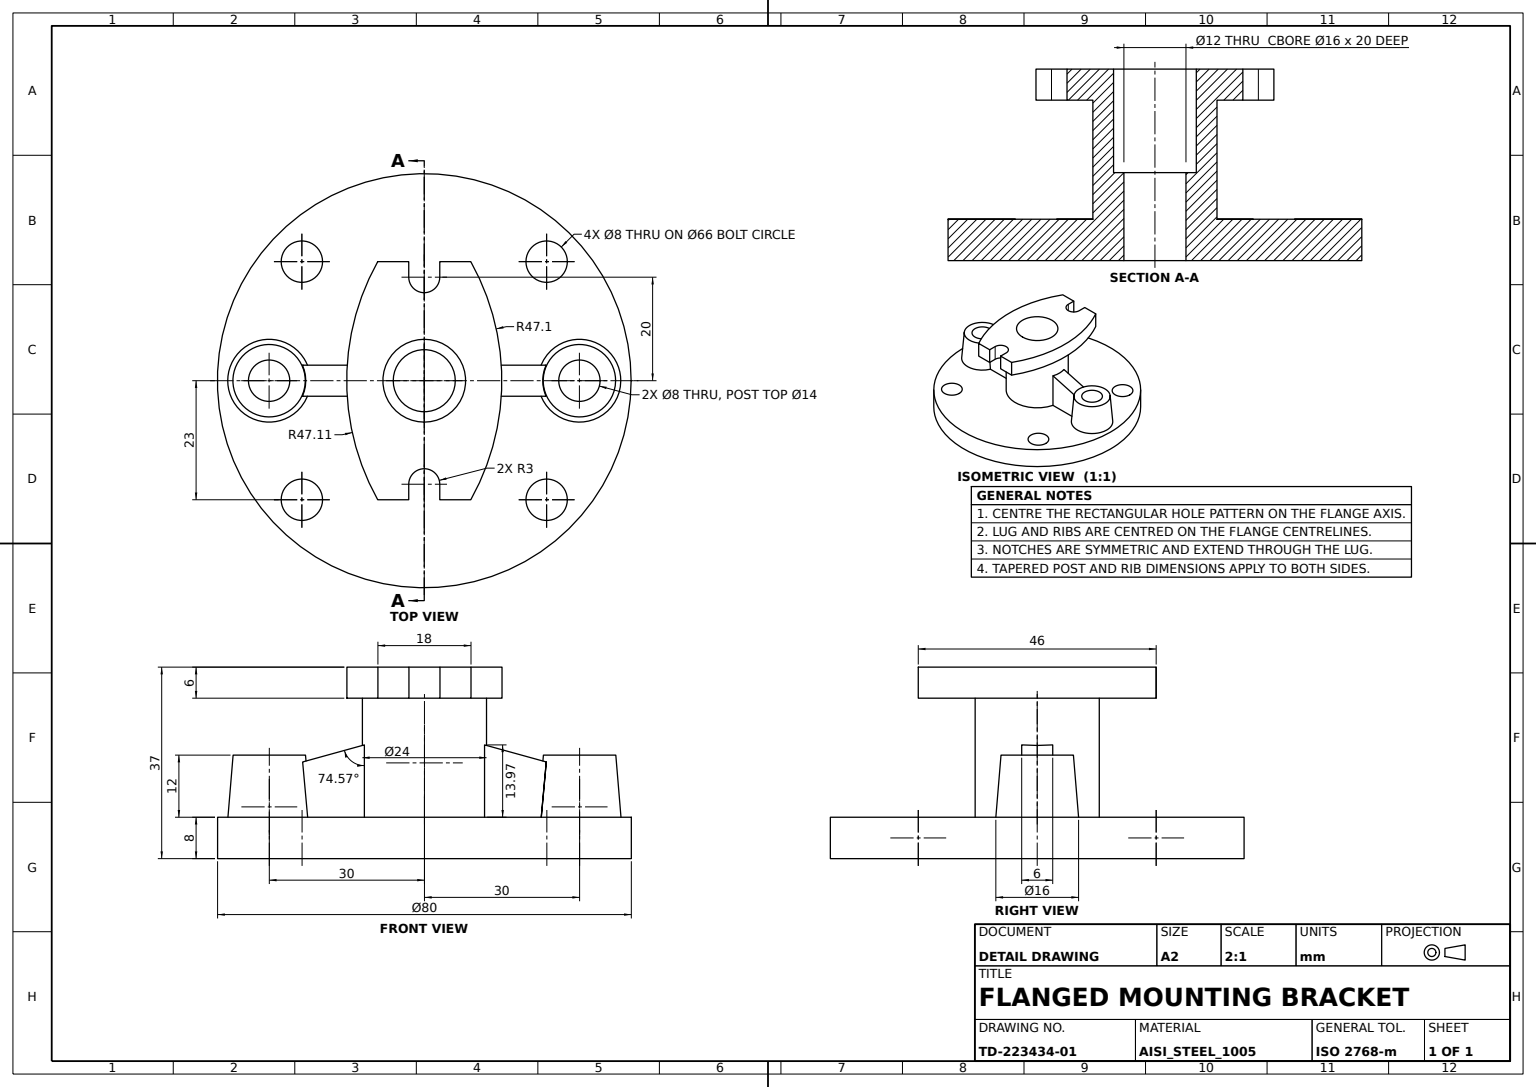
ISO-10303-21;
HEADER;
FILE_DESCRIPTION((''),'2;1');
FILE_NAME('','',(''),(''),'','','');
FILE_SCHEMA(('AUTOMOTIVE_DESIGN'));
ENDSEC;
DATA;
#1=APPLICATION_CONTEXT('');
#2=PRODUCT_CONTEXT('',#1,'mechanical');
#3=PRODUCT('','','',(#2));
#4=PRODUCT_DEFINITION_FORMATION('','',#3);
#5=PRODUCT_DEFINITION_CONTEXT('',#1,'design');
#6=PRODUCT_DEFINITION('','',#4,#5);
#7=PRODUCT_DEFINITION_SHAPE('','',#6);
#8=(LENGTH_UNIT()NAMED_UNIT(*)SI_UNIT(.MILLI.,.METRE.));
#9=(NAMED_UNIT(*)PLANE_ANGLE_UNIT()SI_UNIT($,.RADIAN.));
#10=(NAMED_UNIT(*)SI_UNIT($,.STERADIAN.)SOLID_ANGLE_UNIT());
#11=UNCERTAINTY_MEASURE_WITH_UNIT(LENGTH_MEASURE(0.005),#8,'distance_accuracy_value','');
#12=(GEOMETRIC_REPRESENTATION_CONTEXT(3)GLOBAL_UNCERTAINTY_ASSIGNED_CONTEXT((#11))GLOBAL_UNIT_ASSIGNED_CONTEXT((#8,#9,#10))REPRESENTATION_CONTEXT('',''));
#13=CARTESIAN_POINT('',(11.61895,-3.,21.973992));
#14=VERTEX_POINT('',#13);
#15=CARTESIAN_POINT('',(11.61895,3.,21.973992));
#16=VERTEX_POINT('',#15);
#17=CARTESIAN_POINT('',(0.,0.,25.180795));
#18=DIRECTION('',(0.266050452,0.,0.963959106));
#19=DIRECTION('',(0.963959106,0.,-0.266050452));
#20=AXIS2_PLACEMENT_3D('',#17,#18,#19);
#21=ELLIPSE('',#20,12.448661,12.);
#22=EDGE_CURVE('',#14,#16,#21,.T.);
#23=ORIENTED_EDGE('',*,*,#22,.F.);
#24=CARTESIAN_POINT('',(23.554945,-3.,18.679685));
#25=VERTEX_POINT('',#24);
#26=CARTESIAN_POINT('',(10.87655,-3.,22.178892));
#27=VECTOR('',#19,1000.);
#28=LINE('',#26,#27);
#29=EDGE_CURVE('',#14,#25,#28,.T.);
#30=ORIENTED_EDGE('',*,*,#29,.T.);
#31=CARTESIAN_POINT('',(23.554945,3.,18.679685));
#32=VERTEX_POINT('',#31);
#33=CARTESIAN_POINT('',(22.695172,1.11677,18.91698));
#34=CARTESIAN_POINT('',(22.695241,-1.11692,18.916962));
#35=B_SPLINE_CURVE_WITH_KNOTS('',3,(#31,#33,#34,#24),.UNSPECIFIED.,.F.,.F.,(4,4),(0.,0.006162531),.UNSPECIFIED.);
#36=EDGE_CURVE('',#32,#25,#35,.T.);
#37=ORIENTED_EDGE('',*,*,#36,.F.);
#38=CARTESIAN_POINT('',(10.87655,3.,22.178892));
#39=LINE('',#38,#27);
#40=EDGE_CURVE('',#16,#32,#39,.T.);
#41=ORIENTED_EDGE('',*,*,#40,.F.);
#42=EDGE_LOOP('',(#23,#30,#37,#41));
#43=FACE_BOUND('',#42,.T.);
#44=AXIS2_PLACEMENT_3D('',#26,#18,#19);
#45=PLANE('',#44);
#46=ADVANCED_FACE('',(#43),#45,.T.);
#47=CARTESIAN_POINT('',(0.,-8.,17.));
#48=VERTEX_POINT('',#47);
#49=CARTESIAN_POINT('',(0.,0.,17.));
#50=DIRECTION('',(0.,0.,-1.));
#51=DIRECTION('',(0.,-1.,0.));
#52=AXIS2_PLACEMENT_3D('',#49,#50,#51);
#53=CIRCLE('',#52,8.);
#54=EDGE_CURVE('',#48,#48,#53,.F.);
#55=ORIENTED_EDGE('',*,*,#54,.T.);
#56=EDGE_LOOP('',(#55));
#57=FACE_BOUND('',#56,.T.);
#58=CARTESIAN_POINT('',(-6.,0.,17.));
#59=VERTEX_POINT('',#58);
#60=DIRECTION('',(-1.,0.,0.));
#61=AXIS2_PLACEMENT_3D('',#49,#50,#60);
#62=CIRCLE('',#61,6.);
#63=EDGE_CURVE('',#59,#59,#62,.T.);
#64=ORIENTED_EDGE('',*,*,#63,.T.);
#65=EDGE_LOOP('',(#64));
#66=FACE_BOUND('',#65,.T.);
#67=PLANE('',#61);
#68=ADVANCED_FACE('',(#57,#66),#67,.F.);
#69=CARTESIAN_POINT('',(6.,0.,0.));
#70=VERTEX_POINT('',#69);
#71=CARTESIAN_POINT('',(0.,0.,0.));
#72=DIRECTION('',(1.,0.,0.));
#73=AXIS2_PLACEMENT_3D('',#71,#50,#72);
#74=CIRCLE('',#73,6.);
#75=EDGE_CURVE('',#70,#70,#74,.T.);
#76=ORIENTED_EDGE('',*,*,#75,.F.);
#77=EDGE_LOOP('',(#76));
#78=FACE_BOUND('',#77,.T.);
#79=CARTESIAN_POINT('',(19.664319,23.,0.));
#80=VERTEX_POINT('',#79);
#81=CARTESIAN_POINT('',(23.664319,23.,0.));
#82=AXIS2_PLACEMENT_3D('',#81,#50,#60);
#83=CIRCLE('',#82,4.);
#84=EDGE_CURVE('',#80,#80,#83,.F.);
#85=ORIENTED_EDGE('',*,*,#84,.T.);
#86=EDGE_LOOP('',(#85));
#87=FACE_BOUND('',#86,.T.);
#88=CARTESIAN_POINT('',(-27.664319,-23.,0.));
#89=VERTEX_POINT('',#88);
#90=CARTESIAN_POINT('',(-23.664319,-23.,0.));
#91=AXIS2_PLACEMENT_3D('',#90,#50,#60);
#92=CIRCLE('',#91,4.);
#93=EDGE_CURVE('',#89,#89,#92,.F.);
#94=ORIENTED_EDGE('',*,*,#93,.T.);
#95=EDGE_LOOP('',(#94));
#96=FACE_BOUND('',#95,.T.);
#97=CARTESIAN_POINT('',(26.,0.,0.));
#98=VERTEX_POINT('',#97);
#99=CARTESIAN_POINT('',(30.,0.,0.));
#100=AXIS2_PLACEMENT_3D('',#99,#50,#60);
#101=CIRCLE('',#100,4.);
#102=EDGE_CURVE('',#98,#98,#101,.F.);
#103=ORIENTED_EDGE('',*,*,#102,.T.);
#104=EDGE_LOOP('',(#103));
#105=FACE_BOUND('',#104,.T.);
#106=CARTESIAN_POINT('',(-34.,0.,0.));
#107=VERTEX_POINT('',#106);
#108=CARTESIAN_POINT('',(-30.,0.,0.));
#109=AXIS2_PLACEMENT_3D('',#108,#50,#60);
#110=CIRCLE('',#109,4.);
#111=EDGE_CURVE('',#107,#107,#110,.F.);
#112=ORIENTED_EDGE('',*,*,#111,.T.);
#113=EDGE_LOOP('',(#112));
#114=FACE_BOUND('',#113,.T.);
#115=CARTESIAN_POINT('',(-27.664319,23.,0.));
#116=VERTEX_POINT('',#115);
#117=CARTESIAN_POINT('',(-23.664319,23.,0.));
#118=AXIS2_PLACEMENT_3D('',#117,#50,#60);
#119=CIRCLE('',#118,4.);
#120=EDGE_CURVE('',#116,#116,#119,.F.);
#121=ORIENTED_EDGE('',*,*,#120,.T.);
#122=EDGE_LOOP('',(#121));
#123=FACE_BOUND('',#122,.T.);
#124=CARTESIAN_POINT('',(19.664319,-23.,0.));
#125=VERTEX_POINT('',#124);
#126=CARTESIAN_POINT('',(23.664319,-23.,0.));
#127=AXIS2_PLACEMENT_3D('',#126,#50,#60);
#128=CIRCLE('',#127,4.);
#129=EDGE_CURVE('',#125,#125,#128,.F.);
#130=ORIENTED_EDGE('',*,*,#129,.T.);
#131=EDGE_LOOP('',(#130));
#132=FACE_BOUND('',#131,.T.);
#133=CARTESIAN_POINT('',(40.,0.,0.));
#134=VERTEX_POINT('',#133);
#135=CIRCLE('',#73,40.);
#136=EDGE_CURVE('',#134,#134,#135,.T.);
#137=ORIENTED_EDGE('',*,*,#136,.T.);
#138=EDGE_LOOP('',(#137));
#139=FACE_BOUND('',#138,.T.);
#140=AXIS2_PLACEMENT_3D('',#71,#50,#60);
#141=PLANE('',#140);
#142=ADVANCED_FACE('',(#78,#87,#96,#105,#114,#123,#132,#139),#141,.T.);
#143=ORIENTED_EDGE('',*,*,#75,.T.);
#144=EDGE_LOOP('',(#143));
#145=FACE_BOUND('',#144,.T.);
#146=ORIENTED_EDGE('',*,*,#63,.F.);
#147=EDGE_LOOP('',(#146));
#148=FACE_BOUND('',#147,.T.);
#149=CARTESIAN_POINT('',(0.,0.,20.));
#150=AXIS2_PLACEMENT_3D('',#149,#50,#60);
#151=CYLINDRICAL_SURFACE('',#150,6.);
#152=ADVANCED_FACE('',(#145,#148),#151,.F.);
#153=CARTESIAN_POINT('',(-9.,-23.,37.));
#154=VERTEX_POINT('',#153);
#155=CARTESIAN_POINT('',(-9.,-23.,31.));
#156=VERTEX_POINT('',#155);
#157=VECTOR('',#50,1000.);
#158=LINE('',#153,#157);
#159=EDGE_CURVE('',#154,#156,#158,.T.);
#160=ORIENTED_EDGE('',*,*,#159,.T.);
#161=CARTESIAN_POINT('',(-3.,-23.,31.));
#162=VERTEX_POINT('',#161);
#163=VECTOR('',#72,1000.);
#164=LINE('',#155,#163);
#165=EDGE_CURVE('',#156,#162,#164,.T.);
#166=ORIENTED_EDGE('',*,*,#165,.T.);
#167=CARTESIAN_POINT('',(-3.,-23.,37.));
#168=VERTEX_POINT('',#167);
#169=LINE('',#167,#157);
#170=EDGE_CURVE('',#168,#162,#169,.T.);
#171=ORIENTED_EDGE('',*,*,#170,.F.);
#172=LINE('',#153,#163);
#173=EDGE_CURVE('',#154,#168,#172,.T.);
#174=ORIENTED_EDGE('',*,*,#173,.F.);
#175=EDGE_LOOP('',(#160,#166,#171,#174));
#176=FACE_BOUND('',#175,.T.);
#177=DIRECTION('',(0.,1.,0.));
#178=DIRECTION('',(0.,0.,1.));
#179=AXIS2_PLACEMENT_3D('',#153,#177,#178);
#180=PLANE('',#179);
#181=ADVANCED_FACE('',(#176),#180,.F.);
#182=CARTESIAN_POINT('',(3.,-20.,37.));
#183=VERTEX_POINT('',#182);
#184=CARTESIAN_POINT('',(3.,-20.,31.));
#185=VERTEX_POINT('',#184);
#186=LINE('',#182,#157);
#187=EDGE_CURVE('',#183,#185,#186,.T.);
#188=ORIENTED_EDGE('',*,*,#187,.F.);
#189=CARTESIAN_POINT('',(-3.,-20.,37.));
#190=VERTEX_POINT('',#189);
#191=CARTESIAN_POINT('',(0.,-20.,37.));
#192=AXIS2_PLACEMENT_3D('',#191,#50,#72);
#193=CIRCLE('',#192,3.);
#194=EDGE_CURVE('',#190,#183,#193,.T.);
#195=ORIENTED_EDGE('',*,*,#194,.F.);
#196=CARTESIAN_POINT('',(-3.,-20.,31.));
#197=VERTEX_POINT('',#196);
#198=LINE('',#189,#157);
#199=EDGE_CURVE('',#190,#197,#198,.T.);
#200=ORIENTED_EDGE('',*,*,#199,.T.);
#201=CARTESIAN_POINT('',(0.,-20.,31.));
#202=AXIS2_PLACEMENT_3D('',#201,#50,#72);
#203=CIRCLE('',#202,3.);
#204=EDGE_CURVE('',#197,#185,#203,.T.);
#205=ORIENTED_EDGE('',*,*,#204,.T.);
#206=EDGE_LOOP('',(#188,#195,#200,#205));
#207=FACE_BOUND('',#206,.T.);
#208=AXIS2_PLACEMENT_3D('',#191,#50,#60);
#209=CYLINDRICAL_SURFACE('',#208,3.);
#210=ADVANCED_FACE('',(#207),#209,.F.);
#211=CARTESIAN_POINT('',(34.,0.,20.));
#212=VERTEX_POINT('',#211);
#213=CARTESIAN_POINT('',(30.,0.,20.));
#214=AXIS2_PLACEMENT_3D('',#213,#50,#72);
#215=CIRCLE('',#214,4.);
#216=EDGE_CURVE('',#212,#212,#215,.T.);
#217=ORIENTED_EDGE('',*,*,#216,.F.);
#218=EDGE_LOOP('',(#217));
#219=FACE_BOUND('',#218,.T.);
#220=ORIENTED_EDGE('',*,*,#102,.F.);
#221=EDGE_LOOP('',(#220));
#222=FACE_BOUND('',#221,.T.);
#223=CARTESIAN_POINT('',(30.,0.,-5.));
#224=AXIS2_PLACEMENT_3D('',#223,#178,#72);
#225=CYLINDRICAL_SURFACE('',#224,4.);
#226=ADVANCED_FACE('',(#219,#222),#225,.F.);
#227=CARTESIAN_POINT('',(-11.61895,3.,8.));
#228=VERTEX_POINT('',#227);
#229=CARTESIAN_POINT('',(11.61895,3.,8.));
#230=VERTEX_POINT('',#229);
#231=CARTESIAN_POINT('',(0.,0.,8.));
#232=AXIS2_PLACEMENT_3D('',#231,#50,#72);
#233=CIRCLE('',#232,12.);
#234=EDGE_CURVE('',#228,#230,#233,.T.);
#235=ORIENTED_EDGE('',*,*,#234,.F.);
#236=CARTESIAN_POINT('',(-11.61895,3.,21.973992));
#237=VERTEX_POINT('',#236);
#238=CARTESIAN_POINT('',(-11.61895,3.,31.));
#239=LINE('',#238,#157);
#240=EDGE_CURVE('',#237,#228,#239,.T.);
#241=ORIENTED_EDGE('',*,*,#240,.F.);
#242=CARTESIAN_POINT('',(-11.61895,-3.,21.973992));
#243=VERTEX_POINT('',#242);
#244=DIRECTION('',(0.266050452,0.,-0.963959106));
#245=DIRECTION('',(-0.963959106,0.,-0.266050452));
#246=AXIS2_PLACEMENT_3D('',#17,#244,#245);
#247=ELLIPSE('',#246,12.448661,12.);
#248=EDGE_CURVE('',#243,#237,#247,.T.);
#249=ORIENTED_EDGE('',*,*,#248,.F.);
#250=CARTESIAN_POINT('',(-11.61895,-3.,8.));
#251=VERTEX_POINT('',#250);
#252=CARTESIAN_POINT('',(-11.61895,-3.,31.));
#253=LINE('',#252,#157);
#254=EDGE_CURVE('',#243,#251,#253,.T.);
#255=ORIENTED_EDGE('',*,*,#254,.T.);
#256=CARTESIAN_POINT('',(11.61895,-3.,8.));
#257=VERTEX_POINT('',#256);
#258=EDGE_CURVE('',#257,#251,#233,.T.);
#259=ORIENTED_EDGE('',*,*,#258,.F.);
#260=CARTESIAN_POINT('',(11.61895,-3.,31.));
#261=LINE('',#260,#157);
#262=EDGE_CURVE('',#14,#257,#261,.T.);
#263=ORIENTED_EDGE('',*,*,#262,.F.);
#264=ORIENTED_EDGE('',*,*,#22,.T.);
#265=CARTESIAN_POINT('',(11.61895,3.,31.));
#266=LINE('',#265,#157);
#267=EDGE_CURVE('',#16,#230,#266,.T.);
#268=ORIENTED_EDGE('',*,*,#267,.T.);
#269=EDGE_LOOP('',(#235,#241,#249,#255,#259,#263,#264,#268));
#270=FACE_BOUND('',#269,.T.);
#271=CARTESIAN_POINT('',(12.,0.,31.));
#272=VERTEX_POINT('',#271);
#273=CARTESIAN_POINT('',(0.,0.,31.));
#274=AXIS2_PLACEMENT_3D('',#273,#50,#72);
#275=CIRCLE('',#274,12.);
#276=EDGE_CURVE('',#272,#272,#275,.T.);
#277=ORIENTED_EDGE('',*,*,#276,.T.);
#278=EDGE_LOOP('',(#277));
#279=FACE_BOUND('',#278,.T.);
#280=AXIS2_PLACEMENT_3D('',#273,#50,#60);
#281=CYLINDRICAL_SURFACE('',#280,12.);
#282=ADVANCED_FACE('',(#270,#279),#281,.T.);
#283=CARTESIAN_POINT('',(-22.584112,3.,8.));
#284=VERTEX_POINT('',#283);
#285=CARTESIAN_POINT('',(-23.554945,3.,18.679685));
#286=VERTEX_POINT('',#285);
#287=CARTESIAN_POINT('',(-22.904332,3.,11.560202));
#288=CARTESIAN_POINT('',(-23.227468,3.,15.120143));
#289=B_SPLINE_CURVE_WITH_KNOTS('',3,(#283,#287,#288,#285),.UNSPECIFIED.,.F.,.F.,(4,4),(0.,0.010723723),.UNSPECIFIED.);
#290=EDGE_CURVE('',#284,#286,#289,.T.);
#291=ORIENTED_EDGE('',*,*,#290,.F.);
#292=CARTESIAN_POINT('',(-22.584112,-3.,8.));
#293=VERTEX_POINT('',#292);
#294=CARTESIAN_POINT('',(-22.,0.942809,8.));
#295=CARTESIAN_POINT('',(-22.,-0.942809,8.));
#296=CARTESIAN_POINT('',(-22.342339,-2.980208,8.));
#297=CARTESIAN_POINT('',(-24.174186,-5.825814,8.));
#298=CARTESIAN_POINT('',(-26.545524,-7.352354,8.));
#299=CARTESIAN_POINT('',(-28.547841,-7.914415,8.));
#300=CARTESIAN_POINT('',(-30.,-8.042792,8.));
#301=CARTESIAN_POINT('',(-31.452159,-7.914415,8.));
#302=CARTESIAN_POINT('',(-33.454476,-7.352354,8.));
#303=CARTESIAN_POINT('',(-35.825814,-5.825814,8.));
#304=CARTESIAN_POINT('',(-37.352354,-3.454476,8.));
#305=CARTESIAN_POINT('',(-37.914415,-1.452159,8.));
#306=CARTESIAN_POINT('',(-38.042792,0.,8.));
#307=CARTESIAN_POINT('',(-37.914415,1.452159,8.));
#308=CARTESIAN_POINT('',(-37.352354,3.454476,8.));
#309=CARTESIAN_POINT('',(-35.825814,5.825814,8.));
#310=CARTESIAN_POINT('',(-33.454476,7.352354,8.));
#311=CARTESIAN_POINT('',(-31.452159,7.914415,8.));
#312=CARTESIAN_POINT('',(-30.,8.042792,8.));
#313=CARTESIAN_POINT('',(-28.547841,7.914415,8.));
#314=CARTESIAN_POINT('',(-26.545524,7.352354,8.));
#315=CARTESIAN_POINT('',(-24.174186,5.825814,8.));
#316=CARTESIAN_POINT('',(-22.342339,2.980208,8.));
#317=B_SPLINE_CURVE_WITH_KNOTS('',3,(#294,#295,#296,#297,#298,#299,#300,#301,#302,#303,#304,#305,#306,#307,#308,#309,#310,#311,#312,#313,#314,#315,#316,#294,#295),.UNSPECIFIED.,.T.,.F.,(1,1,2,1,1,1,1,1,1,1,1,1,1,1,1,1,1,1,1,1,1,1,1,1,2,1,1),(-0.125,-0.0625,0.,0.0625,0.125,0.1875,0.21875,0.25,0.28125,0.3125,0.375,0.4375,0.46875,0.5,0.53125,0.5625,0.625,0.6875,0.71875,0.75,0.78125,0.8125,0.875,0.9375,1.,1.0625,1.125),.UNSPECIFIED.);
#318=EDGE_CURVE('',#293,#284,#317,.T.);
#319=ORIENTED_EDGE('',*,*,#318,.F.);
#320=CARTESIAN_POINT('',(-23.554945,-3.,18.679685));
#321=VERTEX_POINT('',#320);
#322=CARTESIAN_POINT('',(-22.904332,-3.,11.560202));
#323=CARTESIAN_POINT('',(-23.227468,-3.,15.120143));
#324=B_SPLINE_CURVE_WITH_KNOTS('',3,(#292,#322,#323,#320),.UNSPECIFIED.,.F.,.F.,(4,4),(0.,0.010723723),.UNSPECIFIED.);
#325=EDGE_CURVE('',#293,#321,#324,.T.);
#326=ORIENTED_EDGE('',*,*,#325,.T.);
#327=CARTESIAN_POINT('',(-22.695061,1.116526,18.917011));
#328=CARTESIAN_POINT('',(-22.695433,-1.117342,18.916908));
#329=B_SPLINE_CURVE_WITH_KNOTS('',3,(#285,#327,#328,#320),.UNSPECIFIED.,.F.,.F.,(4,4),(0.,0.006163327),.UNSPECIFIED.);
#330=EDGE_CURVE('',#286,#321,#329,.T.);
#331=ORIENTED_EDGE('',*,*,#330,.F.);
#332=EDGE_LOOP('',(#291,#319,#326,#331));
#333=FACE_BOUND('',#332,.T.);
#334=CARTESIAN_POINT('',(-23.,0.,20.));
#335=VERTEX_POINT('',#334);
#336=CARTESIAN_POINT('',(-23.,0.824958,20.));
#337=CARTESIAN_POINT('',(-23.,-0.824958,20.));
#338=CARTESIAN_POINT('',(-23.299546,-2.607682,20.));
#339=CARTESIAN_POINT('',(-24.902413,-5.097587,20.));
#340=CARTESIAN_POINT('',(-26.977334,-6.433309,20.));
#341=CARTESIAN_POINT('',(-28.729361,-6.925113,20.));
#342=CARTESIAN_POINT('',(-30.,-7.037443,20.));
#343=CARTESIAN_POINT('',(-31.270639,-6.925113,20.));
#344=CARTESIAN_POINT('',(-33.022666,-6.433309,20.));
#345=CARTESIAN_POINT('',(-35.097587,-5.097587,20.));
#346=CARTESIAN_POINT('',(-36.433309,-3.022666,20.));
#347=CARTESIAN_POINT('',(-36.925113,-1.270639,20.));
#348=CARTESIAN_POINT('',(-37.037443,0.,20.));
#349=CARTESIAN_POINT('',(-36.925113,1.270639,20.));
#350=CARTESIAN_POINT('',(-36.433309,3.022666,20.));
#351=CARTESIAN_POINT('',(-35.097587,5.097587,20.));
#352=CARTESIAN_POINT('',(-33.022666,6.433309,20.));
#353=CARTESIAN_POINT('',(-31.270639,6.925113,20.));
#354=CARTESIAN_POINT('',(-30.,7.037443,20.));
#355=CARTESIAN_POINT('',(-28.729361,6.925113,20.));
#356=CARTESIAN_POINT('',(-26.977334,6.433309,20.));
#357=CARTESIAN_POINT('',(-24.902413,5.097587,20.));
#358=CARTESIAN_POINT('',(-23.299546,2.607682,20.));
#359=B_SPLINE_CURVE_WITH_KNOTS('',3,(#336,#337,#338,#339,#340,#341,#342,#343,#344,#345,#346,#347,#348,#349,#350,#351,#352,#353,#354,#355,#356,#357,#358,#336,#337),.UNSPECIFIED.,.T.,.F.,(1,1,2,1,1,1,1,1,1,1,1,1,1,1,1,1,1,1,1,1,1,1,1,1,2,1,1),(-0.125,-0.0625,0.,0.0625,0.125,0.1875,0.21875,0.25,0.28125,0.3125,0.375,0.4375,0.46875,0.5,0.53125,0.5625,0.625,0.6875,0.71875,0.75,0.78125,0.8125,0.875,0.9375,1.,1.0625,1.125),.UNSPECIFIED.);
#360=EDGE_CURVE('',#335,#335,#359,.F.);
#361=ORIENTED_EDGE('',*,*,#360,.F.);
#362=EDGE_LOOP('',(#361));
#363=FACE_BOUND('',#362,.T.);
#364=CARTESIAN_POINT('',(-22.333333,0.903525,12.));
#365=CARTESIAN_POINT('',(-22.666667,0.864242,16.));
#366=CARTESIAN_POINT('',(-22.333333,-0.903525,12.));
#367=CARTESIAN_POINT('',(-22.666667,-0.864242,16.));
#368=CARTESIAN_POINT('',(-22.661408,-2.856033,12.));
#369=CARTESIAN_POINT('',(-22.980477,-2.731857,16.));
#370=CARTESIAN_POINT('',(-24.416928,-5.583072,12.));
#371=CARTESIAN_POINT('',(-24.65967,-5.34033,16.));
#372=CARTESIAN_POINT('',(-26.689461,-7.046005,12.));
#373=CARTESIAN_POINT('',(-26.833397,-6.739657,16.));
#374=CARTESIAN_POINT('',(-28.608348,-7.584648,12.));
#375=CARTESIAN_POINT('',(-28.668854,-7.254881,16.));
#376=CARTESIAN_POINT('',(-30.,-7.707676,12.));
#377=CARTESIAN_POINT('',(-30.,-7.37256,16.));
#378=CARTESIAN_POINT('',(-31.391652,-7.584648,12.));
#379=CARTESIAN_POINT('',(-31.331146,-7.254881,16.));
#380=CARTESIAN_POINT('',(-33.310539,-7.046005,12.));
#381=CARTESIAN_POINT('',(-33.166603,-6.739657,16.));
#382=CARTESIAN_POINT('',(-35.583072,-5.583072,12.));
#383=CARTESIAN_POINT('',(-35.34033,-5.34033,16.));
#384=CARTESIAN_POINT('',(-37.046005,-3.310539,12.));
#385=CARTESIAN_POINT('',(-36.739657,-3.166603,16.));
#386=CARTESIAN_POINT('',(-37.584648,-1.391652,12.));
#387=CARTESIAN_POINT('',(-37.254881,-1.331146,16.));
#388=CARTESIAN_POINT('',(-37.707676,0.,12.));
#389=CARTESIAN_POINT('',(-37.37256,0.,16.));
#390=CARTESIAN_POINT('',(-37.584648,1.391652,12.));
#391=CARTESIAN_POINT('',(-37.254881,1.331146,16.));
#392=CARTESIAN_POINT('',(-37.046005,3.310539,12.));
#393=CARTESIAN_POINT('',(-36.739657,3.166603,16.));
#394=CARTESIAN_POINT('',(-35.583072,5.583072,12.));
#395=CARTESIAN_POINT('',(-35.34033,5.34033,16.));
#396=CARTESIAN_POINT('',(-33.310539,7.046005,12.));
#397=CARTESIAN_POINT('',(-33.166603,6.739657,16.));
#398=CARTESIAN_POINT('',(-31.391652,7.584648,12.));
#399=CARTESIAN_POINT('',(-31.331146,7.254881,16.));
#400=CARTESIAN_POINT('',(-30.,7.707676,12.));
#401=CARTESIAN_POINT('',(-30.,7.37256,16.));
#402=CARTESIAN_POINT('',(-28.608348,7.584648,12.));
#403=CARTESIAN_POINT('',(-28.668854,7.254881,16.));
#404=CARTESIAN_POINT('',(-26.689461,7.046005,12.));
#405=CARTESIAN_POINT('',(-26.833397,6.739657,16.));
#406=CARTESIAN_POINT('',(-24.416928,5.583072,12.));
#407=CARTESIAN_POINT('',(-24.65967,5.34033,16.));
#408=CARTESIAN_POINT('',(-22.661408,2.856033,12.));
#409=CARTESIAN_POINT('',(-22.980477,2.731857,16.));
#410=B_SPLINE_SURFACE_WITH_KNOTS('',3,3,((#294,#364,#365,#336),(#295,#366,#367,#337),(#296,#368,#369,#338),(#297,#370,#371,#339),(#298,#372,#373,#340),(#299,#374,#375,#341),(#300,#376,#377,#342),(#301,#378,#379,#343),(#302,#380,#381,#344),(#303,#382,#383,#345),(#304,#384,#385,#346),(#305,#386,#387,#347),(#306,#388,#389,#348),(#307,#390,#391,#349),(#308,#392,#393,#350),(#309,#394,#395,#351),(#310,#396,#397,#352),(#311,#398,#399,#353),(#312,#400,#401,#354),(#313,#402,#403,#355),(#314,#404,#405,#356),(#315,#406,#407,#357),(#316,#408,#409,#358),(#294,#364,#365,#336),(#295,#366,#367,#337)),.RULED_SURF.,.T.,.F.,.F.,(1,1,2,1,1,1,1,1,1,1,1,1,1,1,1,1,1,1,1,1,1,1,1,1,2,1,1),(4,4),(-0.125,-0.0625,0.,0.0625,0.125,0.1875,0.21875,0.25,0.28125,0.3125,0.375,0.4375,0.46875,0.5,0.53125,0.5625,0.625,0.6875,0.71875,0.75,0.78125,0.8125,0.875,0.9375,1.,1.0625,1.125),(0.,1.),.UNSPECIFIED.);
#411=ADVANCED_FACE('',(#333,#363),#410,.F.);
#412=CARTESIAN_POINT('',(3.,-23.,31.));
#413=VERTEX_POINT('',#412);
#414=CARTESIAN_POINT('',(9.,-23.,31.));
#415=VERTEX_POINT('',#414);
#416=LINE('',#412,#163);
#417=EDGE_CURVE('',#413,#415,#416,.T.);
#418=ORIENTED_EDGE('',*,*,#417,.T.);
#419=CARTESIAN_POINT('',(9.,-23.,37.));
#420=VERTEX_POINT('',#419);
#421=LINE('',#419,#157);
#422=EDGE_CURVE('',#420,#415,#421,.T.);
#423=ORIENTED_EDGE('',*,*,#422,.F.);
#424=CARTESIAN_POINT('',(3.,-23.,37.));
#425=VERTEX_POINT('',#424);
#426=LINE('',#424,#163);
#427=EDGE_CURVE('',#425,#420,#426,.T.);
#428=ORIENTED_EDGE('',*,*,#427,.F.);
#429=LINE('',#424,#157);
#430=EDGE_CURVE('',#425,#413,#429,.T.);
#431=ORIENTED_EDGE('',*,*,#430,.T.);
#432=EDGE_LOOP('',(#418,#423,#428,#431));
#433=FACE_BOUND('',#432,.T.);
#434=AXIS2_PLACEMENT_3D('',#424,#177,#178);
#435=PLANE('',#434);
#436=ADVANCED_FACE('',(#433),#435,.F.);
#437=VECTOR('',#51,1000.);
#438=LINE('',#184,#437);
#439=EDGE_CURVE('',#185,#413,#438,.T.);
#440=ORIENTED_EDGE('',*,*,#439,.T.);
#441=ORIENTED_EDGE('',*,*,#430,.F.);
#442=LINE('',#182,#437);
#443=EDGE_CURVE('',#183,#425,#442,.T.);
#444=ORIENTED_EDGE('',*,*,#443,.F.);
#445=ORIENTED_EDGE('',*,*,#187,.T.);
#446=EDGE_LOOP('',(#440,#441,#444,#445));
#447=FACE_BOUND('',#446,.T.);
#448=AXIS2_PLACEMENT_3D('',#182,#72,#50);
#449=PLANE('',#448);
#450=ADVANCED_FACE('',(#447),#449,.F.);
#451=CARTESIAN_POINT('',(3.,20.,31.));
#452=VERTEX_POINT('',#451);
#453=CARTESIAN_POINT('',(-3.,20.,31.));
#454=VERTEX_POINT('',#453);
#455=CARTESIAN_POINT('',(0.,20.,31.));
#456=AXIS2_PLACEMENT_3D('',#455,#50,#72);
#457=CIRCLE('',#456,3.);
#458=EDGE_CURVE('',#452,#454,#457,.T.);
#459=ORIENTED_EDGE('',*,*,#458,.T.);
#460=CARTESIAN_POINT('',(-3.,20.,37.));
#461=VERTEX_POINT('',#460);
#462=LINE('',#460,#157);
#463=EDGE_CURVE('',#461,#454,#462,.T.);
#464=ORIENTED_EDGE('',*,*,#463,.F.);
#465=CARTESIAN_POINT('',(3.,20.,37.));
#466=VERTEX_POINT('',#465);
#467=CARTESIAN_POINT('',(0.,20.,37.));
#468=AXIS2_PLACEMENT_3D('',#467,#50,#72);
#469=CIRCLE('',#468,3.);
#470=EDGE_CURVE('',#466,#461,#469,.T.);
#471=ORIENTED_EDGE('',*,*,#470,.F.);
#472=LINE('',#465,#157);
#473=EDGE_CURVE('',#466,#452,#472,.T.);
#474=ORIENTED_EDGE('',*,*,#473,.T.);
#475=EDGE_LOOP('',(#459,#464,#471,#474));
#476=FACE_BOUND('',#475,.T.);
#477=AXIS2_PLACEMENT_3D('',#467,#50,#60);
#478=CYLINDRICAL_SURFACE('',#477,3.);
#479=ADVANCED_FACE('',(#476),#478,.F.);
#480=CARTESIAN_POINT('',(37.,0.,20.));
#481=VERTEX_POINT('',#480);
#482=CARTESIAN_POINT('',(37.,0.824958,20.));
#483=CARTESIAN_POINT('',(37.,-0.824958,20.));
#484=CARTESIAN_POINT('',(36.700454,-2.607682,20.));
#485=CARTESIAN_POINT('',(35.097587,-5.097587,20.));
#486=CARTESIAN_POINT('',(33.022666,-6.433309,20.));
#487=CARTESIAN_POINT('',(31.270639,-6.925113,20.));
#488=CARTESIAN_POINT('',(30.,-7.037443,20.));
#489=CARTESIAN_POINT('',(28.729361,-6.925113,20.));
#490=CARTESIAN_POINT('',(26.977334,-6.433309,20.));
#491=CARTESIAN_POINT('',(24.902413,-5.097587,20.));
#492=CARTESIAN_POINT('',(23.566691,-3.022666,20.));
#493=CARTESIAN_POINT('',(23.074887,-1.270639,20.));
#494=CARTESIAN_POINT('',(22.962557,0.,20.));
#495=CARTESIAN_POINT('',(23.074887,1.270639,20.));
#496=CARTESIAN_POINT('',(23.566691,3.022666,20.));
#497=CARTESIAN_POINT('',(24.902413,5.097587,20.));
#498=CARTESIAN_POINT('',(26.977334,6.433309,20.));
#499=CARTESIAN_POINT('',(28.729361,6.925113,20.));
#500=CARTESIAN_POINT('',(30.,7.037443,20.));
#501=CARTESIAN_POINT('',(31.270639,6.925113,20.));
#502=CARTESIAN_POINT('',(33.022666,6.433309,20.));
#503=CARTESIAN_POINT('',(35.097587,5.097587,20.));
#504=CARTESIAN_POINT('',(36.700454,2.607682,20.));
#505=B_SPLINE_CURVE_WITH_KNOTS('',3,(#482,#483,#484,#485,#486,#487,#488,#489,#490,#491,#492,#493,#494,#495,#496,#497,#498,#499,#500,#501,#502,#503,#504,#482,#483),.UNSPECIFIED.,.T.,.F.,(1,1,2,1,1,1,1,1,1,1,1,1,1,1,1,1,1,1,1,1,1,1,1,1,2,1,1),(-0.125,-0.0625,0.,0.0625,0.125,0.1875,0.21875,0.25,0.28125,0.3125,0.375,0.4375,0.46875,0.5,0.53125,0.5625,0.625,0.6875,0.71875,0.75,0.78125,0.8125,0.875,0.9375,1.,1.0625,1.125),.UNSPECIFIED.);
#506=EDGE_CURVE('',#481,#481,#505,.F.);
#507=ORIENTED_EDGE('',*,*,#506,.F.);
#508=EDGE_LOOP('',(#507));
#509=FACE_BOUND('',#508,.T.);
#510=CARTESIAN_POINT('',(22.584112,3.,8.));
#511=VERTEX_POINT('',#510);
#512=CARTESIAN_POINT('',(22.904332,3.,11.560202));
#513=CARTESIAN_POINT('',(23.227468,3.,15.120143));
#514=B_SPLINE_CURVE_WITH_KNOTS('',3,(#510,#512,#513,#31),.UNSPECIFIED.,.F.,.F.,(4,4),(0.,0.010723723),.UNSPECIFIED.);
#515=EDGE_CURVE('',#511,#32,#514,.T.);
#516=ORIENTED_EDGE('',*,*,#515,.T.);
#517=ORIENTED_EDGE('',*,*,#36,.T.);
#518=CARTESIAN_POINT('',(22.584112,-3.,8.));
#519=VERTEX_POINT('',#518);
#520=CARTESIAN_POINT('',(22.904332,-3.,11.560202));
#521=CARTESIAN_POINT('',(23.227468,-3.,15.120143));
#522=B_SPLINE_CURVE_WITH_KNOTS('',3,(#518,#520,#521,#24),.UNSPECIFIED.,.F.,.F.,(4,4),(0.,0.010723723),.UNSPECIFIED.);
#523=EDGE_CURVE('',#519,#25,#522,.T.);
#524=ORIENTED_EDGE('',*,*,#523,.F.);
#525=CARTESIAN_POINT('',(38.,0.942809,8.));
#526=CARTESIAN_POINT('',(38.,-0.942809,8.));
#527=CARTESIAN_POINT('',(37.657661,-2.980208,8.));
#528=CARTESIAN_POINT('',(35.825814,-5.825814,8.));
#529=CARTESIAN_POINT('',(33.454476,-7.352354,8.));
#530=CARTESIAN_POINT('',(31.452159,-7.914415,8.));
#531=CARTESIAN_POINT('',(30.,-8.042792,8.));
#532=CARTESIAN_POINT('',(28.547841,-7.914415,8.));
#533=CARTESIAN_POINT('',(26.545524,-7.352354,8.));
#534=CARTESIAN_POINT('',(24.174186,-5.825814,8.));
#535=CARTESIAN_POINT('',(22.647646,-3.454476,8.));
#536=CARTESIAN_POINT('',(22.085585,-1.452159,8.));
#537=CARTESIAN_POINT('',(21.957208,0.,8.));
#538=CARTESIAN_POINT('',(22.085585,1.452159,8.));
#539=CARTESIAN_POINT('',(22.647646,3.454476,8.));
#540=CARTESIAN_POINT('',(24.174186,5.825814,8.));
#541=CARTESIAN_POINT('',(26.545524,7.352354,8.));
#542=CARTESIAN_POINT('',(28.547841,7.914415,8.));
#543=CARTESIAN_POINT('',(30.,8.042792,8.));
#544=CARTESIAN_POINT('',(31.452159,7.914415,8.));
#545=CARTESIAN_POINT('',(33.454476,7.352354,8.));
#546=CARTESIAN_POINT('',(35.825814,5.825814,8.));
#547=CARTESIAN_POINT('',(37.657661,2.980208,8.));
#548=B_SPLINE_CURVE_WITH_KNOTS('',3,(#525,#526,#527,#528,#529,#530,#531,#532,#533,#534,#535,#536,#537,#538,#539,#540,#541,#542,#543,#544,#545,#546,#547,#525,#526),.UNSPECIFIED.,.T.,.F.,(1,1,2,1,1,1,1,1,1,1,1,1,1,1,1,1,1,1,1,1,1,1,1,1,2,1,1),(-0.125,-0.0625,0.,0.0625,0.125,0.1875,0.21875,0.25,0.28125,0.3125,0.375,0.4375,0.46875,0.5,0.53125,0.5625,0.625,0.6875,0.71875,0.75,0.78125,0.8125,0.875,0.9375,1.,1.0625,1.125),.UNSPECIFIED.);
#549=EDGE_CURVE('',#511,#519,#548,.T.);
#550=ORIENTED_EDGE('',*,*,#549,.F.);
#551=EDGE_LOOP('',(#516,#517,#524,#550));
#552=FACE_BOUND('',#551,.T.);
#553=CARTESIAN_POINT('',(37.666667,0.903525,12.));
#554=CARTESIAN_POINT('',(37.333333,0.864242,16.));
#555=CARTESIAN_POINT('',(37.666667,-0.903525,12.));
#556=CARTESIAN_POINT('',(37.333333,-0.864242,16.));
#557=CARTESIAN_POINT('',(37.338592,-2.856033,12.));
#558=CARTESIAN_POINT('',(37.019523,-2.731857,16.));
#559=CARTESIAN_POINT('',(35.583072,-5.583072,12.));
#560=CARTESIAN_POINT('',(35.34033,-5.34033,16.));
#561=CARTESIAN_POINT('',(33.310539,-7.046005,12.));
#562=CARTESIAN_POINT('',(33.166603,-6.739657,16.));
#563=CARTESIAN_POINT('',(31.391652,-7.584648,12.));
#564=CARTESIAN_POINT('',(31.331146,-7.254881,16.));
#565=CARTESIAN_POINT('',(30.,-7.707676,12.));
#566=CARTESIAN_POINT('',(30.,-7.37256,16.));
#567=CARTESIAN_POINT('',(28.608348,-7.584648,12.));
#568=CARTESIAN_POINT('',(28.668854,-7.254881,16.));
#569=CARTESIAN_POINT('',(26.689461,-7.046005,12.));
#570=CARTESIAN_POINT('',(26.833397,-6.739657,16.));
#571=CARTESIAN_POINT('',(24.416928,-5.583072,12.));
#572=CARTESIAN_POINT('',(24.65967,-5.34033,16.));
#573=CARTESIAN_POINT('',(22.953995,-3.310539,12.));
#574=CARTESIAN_POINT('',(23.260343,-3.166603,16.));
#575=CARTESIAN_POINT('',(22.415352,-1.391652,12.));
#576=CARTESIAN_POINT('',(22.745119,-1.331146,16.));
#577=CARTESIAN_POINT('',(22.292324,0.,12.));
#578=CARTESIAN_POINT('',(22.62744,0.,16.));
#579=CARTESIAN_POINT('',(22.415352,1.391652,12.));
#580=CARTESIAN_POINT('',(22.745119,1.331146,16.));
#581=CARTESIAN_POINT('',(22.953995,3.310539,12.));
#582=CARTESIAN_POINT('',(23.260343,3.166603,16.));
#583=CARTESIAN_POINT('',(24.416928,5.583072,12.));
#584=CARTESIAN_POINT('',(24.65967,5.34033,16.));
#585=CARTESIAN_POINT('',(26.689461,7.046005,12.));
#586=CARTESIAN_POINT('',(26.833397,6.739657,16.));
#587=CARTESIAN_POINT('',(28.608348,7.584648,12.));
#588=CARTESIAN_POINT('',(28.668854,7.254881,16.));
#589=CARTESIAN_POINT('',(30.,7.707676,12.));
#590=CARTESIAN_POINT('',(30.,7.37256,16.));
#591=CARTESIAN_POINT('',(31.391652,7.584648,12.));
#592=CARTESIAN_POINT('',(31.331146,7.254881,16.));
#593=CARTESIAN_POINT('',(33.310539,7.046005,12.));
#594=CARTESIAN_POINT('',(33.166603,6.739657,16.));
#595=CARTESIAN_POINT('',(35.583072,5.583072,12.));
#596=CARTESIAN_POINT('',(35.34033,5.34033,16.));
#597=CARTESIAN_POINT('',(37.338592,2.856033,12.));
#598=CARTESIAN_POINT('',(37.019523,2.731857,16.));
#599=B_SPLINE_SURFACE_WITH_KNOTS('',3,3,((#525,#553,#554,#482),(#526,#555,#556,#483),(#527,#557,#558,#484),(#528,#559,#560,#485),(#529,#561,#562,#486),(#530,#563,#564,#487),(#531,#565,#566,#488),(#532,#567,#568,#489),(#533,#569,#570,#490),(#534,#571,#572,#491),(#535,#573,#574,#492),(#536,#575,#576,#493),(#537,#577,#578,#494),(#538,#579,#580,#495),(#539,#581,#582,#496),(#540,#583,#584,#497),(#541,#585,#586,#498),(#542,#587,#588,#499),(#543,#589,#590,#500),(#544,#591,#592,#501),(#545,#593,#594,#502),(#546,#595,#596,#503),(#547,#597,#598,#504),(#525,#553,#554,#482),(#526,#555,#556,#483)),.RULED_SURF.,.T.,.F.,.F.,(1,1,2,1,1,1,1,1,1,1,1,1,1,1,1,1,1,1,1,1,1,1,1,1,2,1,1),(4,4),(-0.125,-0.0625,0.,0.0625,0.125,0.1875,0.21875,0.25,0.28125,0.3125,0.375,0.4375,0.46875,0.5,0.53125,0.5625,0.625,0.6875,0.71875,0.75,0.78125,0.8125,0.875,0.9375,1.,1.0625,1.125),(0.,1.),.UNSPECIFIED.);
#600=ADVANCED_FACE('',(#509,#552),#599,.F.);
#601=CARTESIAN_POINT('',(-24.575454,-3.,8.));
#602=LINE('',#601,#163);
#603=EDGE_CURVE('',#293,#251,#602,.T.);
#604=ORIENTED_EDGE('',*,*,#603,.T.);
#605=ORIENTED_EDGE('',*,*,#254,.F.);
#606=CARTESIAN_POINT('',(-10.87655,-3.,22.178892));
#607=VECTOR('',#245,1000.);
#608=LINE('',#606,#607);
#609=EDGE_CURVE('',#243,#321,#608,.T.);
#610=ORIENTED_EDGE('',*,*,#609,.T.);
#611=ORIENTED_EDGE('',*,*,#325,.F.);
#612=EDGE_LOOP('',(#604,#605,#610,#611));
#613=FACE_BOUND('',#612,.T.);
#614=CARTESIAN_POINT('',(0.,-3.,0.));
#615=AXIS2_PLACEMENT_3D('',#614,#51,#50);
#616=PLANE('',#615);
#617=ADVANCED_FACE('',(#613),#616,.T.);
#618=ORIENTED_EDGE('',*,*,#506,.T.);
#619=EDGE_LOOP('',(#618));
#620=FACE_BOUND('',#619,.T.);
#621=ORIENTED_EDGE('',*,*,#216,.T.);
#622=EDGE_LOOP('',(#621));
#623=FACE_BOUND('',#622,.T.);
#624=AXIS2_PLACEMENT_3D('',#213,#178,#177);
#625=PLANE('',#624);
#626=ADVANCED_FACE('',(#620,#623),#625,.T.);
#627=ORIENTED_EDGE('',*,*,#93,.F.);
#628=EDGE_LOOP('',(#627));
#629=FACE_BOUND('',#628,.T.);
#630=CARTESIAN_POINT('',(-19.664319,-23.,8.));
#631=VERTEX_POINT('',#630);
#632=CARTESIAN_POINT('',(-23.664319,-23.,8.));
#633=AXIS2_PLACEMENT_3D('',#632,#50,#72);
#634=CIRCLE('',#633,4.);
#635=EDGE_CURVE('',#631,#631,#634,.T.);
#636=ORIENTED_EDGE('',*,*,#635,.F.);
#637=EDGE_LOOP('',(#636));
#638=FACE_BOUND('',#637,.T.);
#639=CARTESIAN_POINT('',(-23.664319,-23.,-2.));
#640=AXIS2_PLACEMENT_3D('',#639,#178,#72);
#641=CYLINDRICAL_SURFACE('',#640,4.);
#642=ADVANCED_FACE('',(#629,#638),#641,.F.);
#643=CARTESIAN_POINT('',(3.,23.,37.));
#644=VERTEX_POINT('',#643);
#645=CARTESIAN_POINT('',(3.,23.,31.));
#646=VERTEX_POINT('',#645);
#647=LINE('',#643,#157);
#648=EDGE_CURVE('',#644,#646,#647,.T.);
#649=ORIENTED_EDGE('',*,*,#648,.F.);
#650=CARTESIAN_POINT('',(9.,23.,37.));
#651=VERTEX_POINT('',#650);
#652=VECTOR('',#60,1000.);
#653=LINE('',#650,#652);
#654=EDGE_CURVE('',#651,#644,#653,.T.);
#655=ORIENTED_EDGE('',*,*,#654,.F.);
#656=CARTESIAN_POINT('',(9.,23.,31.));
#657=VERTEX_POINT('',#656);
#658=LINE('',#650,#157);
#659=EDGE_CURVE('',#651,#657,#658,.T.);
#660=ORIENTED_EDGE('',*,*,#659,.T.);
#661=LINE('',#656,#652);
#662=EDGE_CURVE('',#657,#646,#661,.T.);
#663=ORIENTED_EDGE('',*,*,#662,.T.);
#664=EDGE_LOOP('',(#649,#655,#660,#663));
#665=FACE_BOUND('',#664,.T.);
#666=AXIS2_PLACEMENT_3D('',#650,#51,#50);
#667=PLANE('',#666);
#668=ADVANCED_FACE('',(#665),#667,.F.);
#669=LINE('',#645,#437);
#670=EDGE_CURVE('',#646,#452,#669,.T.);
#671=ORIENTED_EDGE('',*,*,#670,.T.);
#672=ORIENTED_EDGE('',*,*,#473,.F.);
#673=LINE('',#643,#437);
#674=EDGE_CURVE('',#644,#466,#673,.T.);
#675=ORIENTED_EDGE('',*,*,#674,.F.);
#676=ORIENTED_EDGE('',*,*,#648,.T.);
#677=EDGE_LOOP('',(#671,#672,#675,#676));
#678=FACE_BOUND('',#677,.T.);
#679=AXIS2_PLACEMENT_3D('',#643,#72,#50);
#680=PLANE('',#679);
#681=ADVANCED_FACE('',(#678),#680,.F.);
#682=CARTESIAN_POINT('',(40.,0.,8.));
#683=VERTEX_POINT('',#682);
#684=CIRCLE('',#232,40.);
#685=EDGE_CURVE('',#683,#683,#684,.T.);
#686=ORIENTED_EDGE('',*,*,#685,.F.);
#687=EDGE_LOOP('',(#686));
#688=FACE_BOUND('',#687,.T.);
#689=CARTESIAN_POINT('',(27.664319,-23.,8.));
#690=VERTEX_POINT('',#689);
#691=CARTESIAN_POINT('',(23.664319,-23.,8.));
#692=AXIS2_PLACEMENT_3D('',#691,#50,#72);
#693=CIRCLE('',#692,4.);
#694=EDGE_CURVE('',#690,#690,#693,.T.);
#695=ORIENTED_EDGE('',*,*,#694,.T.);
#696=EDGE_LOOP('',(#695));
#697=FACE_BOUND('',#696,.T.);
#698=ORIENTED_EDGE('',*,*,#635,.T.);
#699=EDGE_LOOP('',(#698));
#700=FACE_BOUND('',#699,.T.);
#701=CARTESIAN_POINT('',(27.664319,23.,8.));
#702=VERTEX_POINT('',#701);
#703=CARTESIAN_POINT('',(23.664319,23.,8.));
#704=AXIS2_PLACEMENT_3D('',#703,#50,#72);
#705=CIRCLE('',#704,4.);
#706=EDGE_CURVE('',#702,#702,#705,.T.);
#707=ORIENTED_EDGE('',*,*,#706,.T.);
#708=EDGE_LOOP('',(#707));
#709=FACE_BOUND('',#708,.T.);
#710=CARTESIAN_POINT('',(-19.664319,23.,8.));
#711=VERTEX_POINT('',#710);
#712=CARTESIAN_POINT('',(-23.664319,23.,8.));
#713=AXIS2_PLACEMENT_3D('',#712,#50,#72);
#714=CIRCLE('',#713,4.);
#715=EDGE_CURVE('',#711,#711,#714,.T.);
#716=ORIENTED_EDGE('',*,*,#715,.T.);
#717=EDGE_LOOP('',(#716));
#718=FACE_BOUND('',#717,.T.);
#719=ORIENTED_EDGE('',*,*,#549,.T.);
#720=CARTESIAN_POINT('',(24.575454,-3.,8.));
#721=LINE('',#720,#652);
#722=EDGE_CURVE('',#519,#257,#721,.T.);
#723=ORIENTED_EDGE('',*,*,#722,.T.);
#724=ORIENTED_EDGE('',*,*,#258,.T.);
#725=ORIENTED_EDGE('',*,*,#603,.F.);
#726=ORIENTED_EDGE('',*,*,#318,.T.);
#727=CARTESIAN_POINT('',(-24.575454,3.,8.));
#728=LINE('',#727,#163);
#729=EDGE_CURVE('',#284,#228,#728,.T.);
#730=ORIENTED_EDGE('',*,*,#729,.T.);
#731=ORIENTED_EDGE('',*,*,#234,.T.);
#732=CARTESIAN_POINT('',(24.575454,3.,8.));
#733=LINE('',#732,#652);
#734=EDGE_CURVE('',#511,#230,#733,.T.);
#735=ORIENTED_EDGE('',*,*,#734,.F.);
#736=EDGE_LOOP('',(#719,#723,#724,#725,#726,#730,#731,#735));
#737=FACE_BOUND('',#736,.T.);
#738=AXIS2_PLACEMENT_3D('',#231,#50,#60);
#739=PLANE('',#738);
#740=ADVANCED_FACE('',(#688,#697,#700,#709,#718,#737),#739,.F.);
#741=ORIENTED_EDGE('',*,*,#54,.F.);
#742=EDGE_LOOP('',(#741));
#743=FACE_BOUND('',#742,.T.);
#744=CARTESIAN_POINT('',(0.,-8.,37.));
#745=VERTEX_POINT('',#744);
#746=CARTESIAN_POINT('',(0.,0.,37.));
#747=AXIS2_PLACEMENT_3D('',#746,#50,#51);
#748=CIRCLE('',#747,8.);
#749=EDGE_CURVE('',#745,#745,#748,.T.);
#750=ORIENTED_EDGE('',*,*,#749,.F.);
#751=EDGE_LOOP('',(#750));
#752=FACE_BOUND('',#751,.T.);
#753=AXIS2_PLACEMENT_3D('',#49,#178,#72);
#754=CYLINDRICAL_SURFACE('',#753,8.);
#755=ADVANCED_FACE('',(#743,#752),#754,.F.);
#756=ORIENTED_EDGE('',*,*,#120,.F.);
#757=EDGE_LOOP('',(#756));
#758=FACE_BOUND('',#757,.T.);
#759=ORIENTED_EDGE('',*,*,#715,.F.);
#760=EDGE_LOOP('',(#759));
#761=FACE_BOUND('',#760,.T.);
#762=CARTESIAN_POINT('',(-23.664319,23.,-2.));
#763=AXIS2_PLACEMENT_3D('',#762,#178,#72);
#764=CYLINDRICAL_SURFACE('',#763,4.);
#765=ADVANCED_FACE('',(#758,#761),#764,.F.);
#766=ORIENTED_EDGE('',*,*,#729,.F.);
#767=ORIENTED_EDGE('',*,*,#290,.T.);
#768=CARTESIAN_POINT('',(-10.87655,3.,22.178892));
#769=LINE('',#768,#607);
#770=EDGE_CURVE('',#237,#286,#769,.T.);
#771=ORIENTED_EDGE('',*,*,#770,.F.);
#772=ORIENTED_EDGE('',*,*,#240,.T.);
#773=EDGE_LOOP('',(#766,#767,#771,#772));
#774=FACE_BOUND('',#773,.T.);
#775=CARTESIAN_POINT('',(0.,3.,0.));
#776=AXIS2_PLACEMENT_3D('',#775,#51,#50);
#777=PLANE('',#776);
#778=ADVANCED_FACE('',(#774),#777,.F.);
#779=ORIENTED_EDGE('',*,*,#262,.T.);
#780=ORIENTED_EDGE('',*,*,#722,.F.);
#781=ORIENTED_EDGE('',*,*,#523,.T.);
#782=ORIENTED_EDGE('',*,*,#29,.F.);
#783=EDGE_LOOP('',(#779,#780,#781,#782));
#784=FACE_BOUND('',#783,.T.);
#785=AXIS2_PLACEMENT_3D('',#614,#177,#178);
#786=PLANE('',#785);
#787=ADVANCED_FACE('',(#784),#786,.F.);
#788=ORIENTED_EDGE('',*,*,#40,.T.);
#789=ORIENTED_EDGE('',*,*,#515,.F.);
#790=ORIENTED_EDGE('',*,*,#734,.T.);
#791=ORIENTED_EDGE('',*,*,#267,.F.);
#792=EDGE_LOOP('',(#788,#789,#790,#791));
#793=FACE_BOUND('',#792,.T.);
#794=AXIS2_PLACEMENT_3D('',#775,#177,#178);
#795=PLANE('',#794);
#796=ADVANCED_FACE('',(#793),#795,.T.);
#797=ORIENTED_EDGE('',*,*,#84,.F.);
#798=EDGE_LOOP('',(#797));
#799=FACE_BOUND('',#798,.T.);
#800=ORIENTED_EDGE('',*,*,#706,.F.);
#801=EDGE_LOOP('',(#800));
#802=FACE_BOUND('',#801,.T.);
#803=CARTESIAN_POINT('',(23.664319,23.,-2.));
#804=AXIS2_PLACEMENT_3D('',#803,#178,#72);
#805=CYLINDRICAL_SURFACE('',#804,4.);
#806=ADVANCED_FACE('',(#799,#802),#805,.F.);
#807=ORIENTED_EDGE('',*,*,#694,.F.);
#808=EDGE_LOOP('',(#807));
#809=FACE_BOUND('',#808,.T.);
#810=ORIENTED_EDGE('',*,*,#129,.F.);
#811=EDGE_LOOP('',(#810));
#812=FACE_BOUND('',#811,.T.);
#813=CARTESIAN_POINT('',(23.664319,-23.,-2.));
#814=AXIS2_PLACEMENT_3D('',#813,#178,#72);
#815=CYLINDRICAL_SURFACE('',#814,4.);
#816=ADVANCED_FACE('',(#809,#812),#815,.F.);
#817=CARTESIAN_POINT('',(-9.,23.,37.));
#818=VERTEX_POINT('',#817);
#819=CARTESIAN_POINT('',(-9.,23.,31.));
#820=VERTEX_POINT('',#819);
#821=LINE('',#817,#157);
#822=EDGE_CURVE('',#818,#820,#821,.T.);
#823=ORIENTED_EDGE('',*,*,#822,.F.);
#824=CARTESIAN_POINT('',(-3.,23.,37.));
#825=VERTEX_POINT('',#824);
#826=LINE('',#824,#652);
#827=EDGE_CURVE('',#825,#818,#826,.T.);
#828=ORIENTED_EDGE('',*,*,#827,.F.);
#829=CARTESIAN_POINT('',(-3.,23.,31.));
#830=VERTEX_POINT('',#829);
#831=LINE('',#824,#157);
#832=EDGE_CURVE('',#825,#830,#831,.T.);
#833=ORIENTED_EDGE('',*,*,#832,.T.);
#834=LINE('',#829,#652);
#835=EDGE_CURVE('',#830,#820,#834,.T.);
#836=ORIENTED_EDGE('',*,*,#835,.T.);
#837=EDGE_LOOP('',(#823,#828,#833,#836));
#838=FACE_BOUND('',#837,.T.);
#839=AXIS2_PLACEMENT_3D('',#824,#51,#50);
#840=PLANE('',#839);
#841=ADVANCED_FACE('',(#838),#840,.F.);
#842=CARTESIAN_POINT('',(-32.105643,0.,37.));
#843=AXIS2_PLACEMENT_3D('',#842,#178,#72);
#844=CIRCLE('',#843,47.102801);
#845=EDGE_CURVE('',#420,#651,#844,.T.);
#846=ORIENTED_EDGE('',*,*,#845,.F.);
#847=ORIENTED_EDGE('',*,*,#422,.T.);
#848=CARTESIAN_POINT('',(-32.105643,0.,31.));
#849=AXIS2_PLACEMENT_3D('',#848,#178,#72);
#850=CIRCLE('',#849,47.102801);
#851=EDGE_CURVE('',#415,#657,#850,.T.);
#852=ORIENTED_EDGE('',*,*,#851,.T.);
#853=ORIENTED_EDGE('',*,*,#659,.F.);
#854=EDGE_LOOP('',(#846,#847,#852,#853));
#855=FACE_BOUND('',#854,.T.);
#856=AXIS2_PLACEMENT_3D('',#842,#50,#60);
#857=CYLINDRICAL_SURFACE('',#856,47.102801);
#858=ADVANCED_FACE('',(#855),#857,.T.);
#859=CARTESIAN_POINT('',(32.110792,0.,37.));
#860=AXIS2_PLACEMENT_3D('',#859,#178,#72);
#861=CIRCLE('',#860,47.107295);
#862=EDGE_CURVE('',#818,#154,#861,.T.);
#863=ORIENTED_EDGE('',*,*,#862,.F.);
#864=ORIENTED_EDGE('',*,*,#822,.T.);
#865=CARTESIAN_POINT('',(32.110792,0.,31.));
#866=AXIS2_PLACEMENT_3D('',#865,#178,#72);
#867=CIRCLE('',#866,47.107295);
#868=EDGE_CURVE('',#820,#156,#867,.T.);
#869=ORIENTED_EDGE('',*,*,#868,.T.);
#870=ORIENTED_EDGE('',*,*,#159,.F.);
#871=EDGE_LOOP('',(#863,#864,#869,#870));
#872=FACE_BOUND('',#871,.T.);
#873=AXIS2_PLACEMENT_3D('',#859,#50,#60);
#874=CYLINDRICAL_SURFACE('',#873,47.107295);
#875=ADVANCED_FACE('',(#872),#874,.T.);
#876=ORIENTED_EDGE('',*,*,#136,.F.);
#877=EDGE_LOOP('',(#876));
#878=FACE_BOUND('',#877,.T.);
#879=ORIENTED_EDGE('',*,*,#685,.T.);
#880=EDGE_LOOP('',(#879));
#881=FACE_BOUND('',#880,.T.);
#882=CYLINDRICAL_SURFACE('',#738,40.);
#883=ADVANCED_FACE('',(#878,#881),#882,.T.);
#884=ORIENTED_EDGE('',*,*,#662,.F.);
#885=ORIENTED_EDGE('',*,*,#851,.F.);
#886=ORIENTED_EDGE('',*,*,#417,.F.);
#887=ORIENTED_EDGE('',*,*,#439,.F.);
#888=ORIENTED_EDGE('',*,*,#204,.F.);
#889=VECTOR('',#177,1000.);
#890=LINE('',#161,#889);
#891=EDGE_CURVE('',#162,#197,#890,.T.);
#892=ORIENTED_EDGE('',*,*,#891,.F.);
#893=ORIENTED_EDGE('',*,*,#165,.F.);
#894=ORIENTED_EDGE('',*,*,#868,.F.);
#895=ORIENTED_EDGE('',*,*,#835,.F.);
#896=LINE('',#453,#889);
#897=EDGE_CURVE('',#454,#830,#896,.T.);
#898=ORIENTED_EDGE('',*,*,#897,.F.);
#899=ORIENTED_EDGE('',*,*,#458,.F.);
#900=ORIENTED_EDGE('',*,*,#670,.F.);
#901=EDGE_LOOP('',(#884,#885,#886,#887,#888,#892,#893,#894,#895,#898,#899,#900));
#902=FACE_BOUND('',#901,.T.);
#903=ORIENTED_EDGE('',*,*,#276,.F.);
#904=EDGE_LOOP('',(#903));
#905=FACE_BOUND('',#904,.T.);
#906=PLANE('',#866);
#907=ADVANCED_FACE('',(#902,#905),#906,.F.);
#908=LINE('',#460,#889);
#909=EDGE_CURVE('',#461,#825,#908,.T.);
#910=ORIENTED_EDGE('',*,*,#909,.F.);
#911=ORIENTED_EDGE('',*,*,#463,.T.);
#912=ORIENTED_EDGE('',*,*,#897,.T.);
#913=ORIENTED_EDGE('',*,*,#832,.F.);
#914=EDGE_LOOP('',(#910,#911,#912,#913));
#915=FACE_BOUND('',#914,.T.);
#916=AXIS2_PLACEMENT_3D('',#460,#60,#178);
#917=PLANE('',#916);
#918=ADVANCED_FACE('',(#915),#917,.F.);
#919=ORIENTED_EDGE('',*,*,#770,.T.);
#920=ORIENTED_EDGE('',*,*,#330,.T.);
#921=ORIENTED_EDGE('',*,*,#609,.F.);
#922=ORIENTED_EDGE('',*,*,#248,.T.);
#923=EDGE_LOOP('',(#919,#920,#921,#922));
#924=FACE_BOUND('',#923,.T.);
#925=AXIS2_PLACEMENT_3D('',#606,#244,#245);
#926=PLANE('',#925);
#927=ADVANCED_FACE('',(#924),#926,.F.);
#928=CARTESIAN_POINT('',(-26.,0.,20.));
#929=VERTEX_POINT('',#928);
#930=CARTESIAN_POINT('',(-30.,0.,20.));
#931=AXIS2_PLACEMENT_3D('',#930,#50,#72);
#932=CIRCLE('',#931,4.);
#933=EDGE_CURVE('',#929,#929,#932,.T.);
#934=ORIENTED_EDGE('',*,*,#933,.F.);
#935=EDGE_LOOP('',(#934));
#936=FACE_BOUND('',#935,.T.);
#937=ORIENTED_EDGE('',*,*,#111,.F.);
#938=EDGE_LOOP('',(#937));
#939=FACE_BOUND('',#938,.T.);
#940=CARTESIAN_POINT('',(-30.,0.,-5.));
#941=AXIS2_PLACEMENT_3D('',#940,#178,#72);
#942=CYLINDRICAL_SURFACE('',#941,4.);
#943=ADVANCED_FACE('',(#936,#939),#942,.F.);
#944=ORIENTED_EDGE('',*,*,#443,.T.);
#945=ORIENTED_EDGE('',*,*,#427,.T.);
#946=ORIENTED_EDGE('',*,*,#845,.T.);
#947=ORIENTED_EDGE('',*,*,#654,.T.);
#948=ORIENTED_EDGE('',*,*,#674,.T.);
#949=ORIENTED_EDGE('',*,*,#470,.T.);
#950=ORIENTED_EDGE('',*,*,#909,.T.);
#951=ORIENTED_EDGE('',*,*,#827,.T.);
#952=ORIENTED_EDGE('',*,*,#862,.T.);
#953=ORIENTED_EDGE('',*,*,#173,.T.);
#954=LINE('',#167,#889);
#955=EDGE_CURVE('',#168,#190,#954,.T.);
#956=ORIENTED_EDGE('',*,*,#955,.T.);
#957=ORIENTED_EDGE('',*,*,#194,.T.);
#958=EDGE_LOOP('',(#944,#945,#946,#947,#948,#949,#950,#951,#952,#953,#956,#957));
#959=FACE_BOUND('',#958,.T.);
#960=ORIENTED_EDGE('',*,*,#749,.T.);
#961=EDGE_LOOP('',(#960));
#962=FACE_BOUND('',#961,.T.);
#963=PLANE('',#860);
#964=ADVANCED_FACE('',(#959,#962),#963,.T.);
#965=ORIENTED_EDGE('',*,*,#170,.T.);
#966=ORIENTED_EDGE('',*,*,#891,.T.);
#967=ORIENTED_EDGE('',*,*,#199,.F.);
#968=ORIENTED_EDGE('',*,*,#955,.F.);
#969=EDGE_LOOP('',(#965,#966,#967,#968));
#970=FACE_BOUND('',#969,.T.);
#971=AXIS2_PLACEMENT_3D('',#167,#60,#178);
#972=PLANE('',#971);
#973=ADVANCED_FACE('',(#970),#972,.F.);
#974=ORIENTED_EDGE('',*,*,#933,.T.);
#975=EDGE_LOOP('',(#974));
#976=FACE_BOUND('',#975,.T.);
#977=ORIENTED_EDGE('',*,*,#360,.T.);
#978=EDGE_LOOP('',(#977));
#979=FACE_BOUND('',#978,.T.);
#980=AXIS2_PLACEMENT_3D('',#930,#178,#177);
#981=PLANE('',#980);
#982=ADVANCED_FACE('',(#976,#979),#981,.T.);
#983=CLOSED_SHELL('',(#46,#68,#142,#152,#181,#210,#226,#282,#411,#436,#450,#479,#600,#617,#626,#642,#668,#681,#740,#755,#765,#778,#787,#796,#806,#816,#841,#858,#875,#883,#907,#918,#927,#943,#964,#973,#982));
#984=MANIFOLD_SOLID_BREP('',#983);
#985=ADVANCED_BREP_SHAPE_REPRESENTATION('',(#984),#12);
#986=SHAPE_DEFINITION_REPRESENTATION(#7,#985);
ENDSEC;
END-ISO-10303-21;
